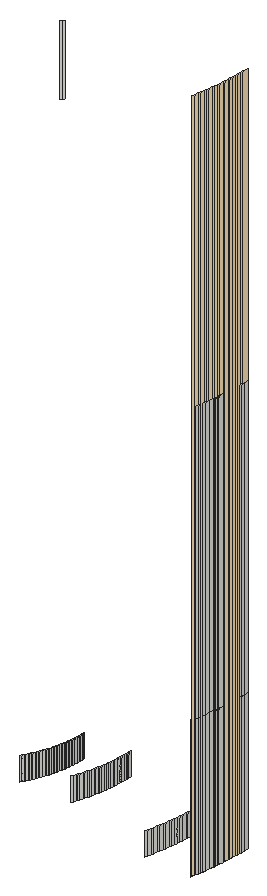
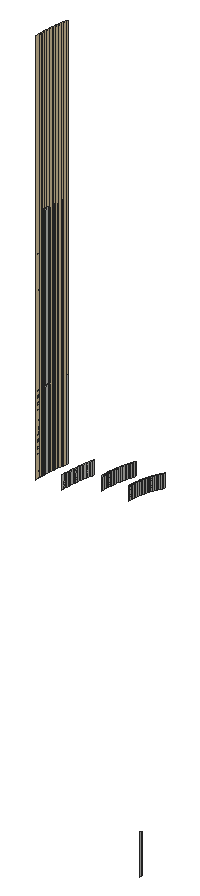
# SketchUp Ruby script. Lengths in inches.
U = 1.inch
M = Sketchup.active_model
def pt(a) = Geom::Point3d.new(a.map { |v| v * U })
def face(e, loops, mat)
  f = e.add_face(loops[0].map { |a| pt(a) })
  loops[1..].each { |l| e.add_face(l.map { |a| pt(a) }).erase! }
  f.material = f.back_material = mat if mat
  f
end
# faces: each face lists its corners as indices into pts; further lists are holes
def faces(e, pts, list, mat = nil) = list.each { |f| face(e, (f[0].is_a?(Array) ? f : [f]).map { |l| l.map { |i| pts[i] } }, mat) }
# xy, xz, yz: faces in a plane at the given z, y or x. An outline is a flat list of corners, or four numbers for a rectangle; further outlines are holes
def ring(l) = l.size == 4 ? [[l[0], l[1]], [l[2], l[1]], [l[2], l[3]], [l[0], l[3]]] : l.each_slice(2).to_a
def flat(e, list, mat, &to3) = list.each { |f| face(e, (f[0].is_a?(Array) ? f : [f]).map { |l| ring(l).map { |u, v| to3.(u, v) } }, mat) }
def xy(e, z, list, mat = nil) = flat(e, list, mat) { |x, y| [x, y, z] }
def xz(e, y, list, mat = nil) = flat(e, list, mat) { |x, z| [x, y, z] }
def yz(e, x, list, mat = nil) = flat(e, list, mat) { |y, z| [x, y, z] }
def lines(e, pts, list) = list.each { |a, b| e.add_line(pt(pts[a]), pt(pts[b])) }
# prism: a flat outline (further loops are holes) pulled along v
def prism(e, loops, v, mat = nil)
  f = face(e, loops, mat); d = Geom::Vector3d.new(v.map { |x| x * U })
  f.pushpull(f.normal.samedirection?(d) ? d.length : -d.length)
end
def box(e, o, s, mat = nil) = prism(e, [[o, [o[0] + s[0], o[1], o[2]], [o[0] + s[0], o[1] + s[1], o[2]], [o[0], o[1] + s[1], o[2]]]], [0, 0, s[2]], mat)
def at(x, y, z, deg = 0) = Geom::Transformation.translation(pt([x, y, z])) * Geom::Transformation.rotation(ORIGIN, Z_AXIS, deg.degrees)
def axes(o, x, y, z) = Geom::Transformation.new([*x, 0, *y, 0, *z, 0, *pt(o).to_a, 1])
def part(name) = M.definitions.add(name)
# library, detail: a bought-in or finely detailed component or shape, given as its bounding box
def library(name, o, s) = part(name).tap { |d| box(d.entities, o, s) }
def detail(e, o, s) = box(e.add_group.entities, o, s)
def put(e, d, t, mat = nil) = e.add_instance(d, t).tap { |i| i.material = mat if mat }
def group(e, t, mat = nil) = e.add_group.tap { |g| g.transformation = t; g.material = mat if mat }.entities
root = M.entities
M.materials.add("1026 AP 7946 SUNNY SIDE UP").color = [254, 231, 186]
yz(root,181.97,[[238.41,247,238.48,248]])
yz(root,181.98,[[238.54,247,238.61,248]])
yz(root,181.99,[[238.67,247,238.74,248]])
yz(root,182,[[238.8,247,238.87,248],[238.87,247,238.93,248],[238.93,247,239,248]])
yz(root,183.99,[[238.54,247,238.63,248],[238.63,247,238.73,248]])
yz(root,184,[[238.82,247,238.91,248],[238.91,247,239,248]])
yz(root,186.99,[[238.48,246,238.61,247]])
yz(root,187,[[238.74,246,238.87,247],[238.87,246,239,247]])
yz(root,188.98,[[238.25,246,238.37,276]],"1026 AP 7946 SUNNY SIDE UP")
yz(root,188.99,[[238.5,246,238.625,276]],"1026 AP 7946 SUNNY SIDE UP")
yz(root,189,[[238.6875,246,238.84,252],[238.84,246,239,252],[238.6875,252,238.84,264],[238.84,252,239,264]])
yz(root,189,[[238.75,246,239,276]],"1026 AP 7946 SUNNY SIDE UP")
p = [[186.69,236.54,246],[186.66,236.41,246],[186.66,236.41,247],[186.69,236.54,247],[188.74,236.51,252],[188.7,236.35,252],
  [188.7,236.35,246],[188.74,236.51,246],[188.74,236.51,246],[188.71,236.38,246],[188.71,236.38,276],[188.74,236.51,276],
  [186.72,236.67,246],[186.72,236.67,247],[188.77,236.66,252],[188.77,236.66,246],[188.76,236.63,246],[188.76,236.63,276],
  [188.79,236.75,246],[188.79,236.75,276],[186.75,236.79,246],[186.75,236.79,247],[188.8,236.8125,252],[188.8,236.8125,246],
  [186.78,236.92,246],[186.78,236.92,247],[188.83,236.97,252],[188.83,236.97,246],[188.81,236.875,246],[188.81,236.875,276],
  [186.81,237.05,246],[186.81,237.05,247],[188.83,237,246],[188.83,237,276],[186.83,237.18,246],[186.83,237.18,247],
  [188.85,237.12,252],[188.85,237.12,246],[188.85,237.12,246],[188.85,237.12,276],[188.875,237.28,252],[188.875,237.28,246],
  [188.87,237.25,246],[188.87,237.25,276],[186.86,237.31,246],[186.86,237.31,247],[188.89,237.37,246],[188.89,237.37,276],
  [186.875,237.4375,246],[186.875,237.4375,247],[188.9,237.43,252],[188.9,237.43,246],[186.9,237.57,246],[186.9,237.57,247],
  [188.92,237.59,252],[188.92,237.59,246],[188.91,237.5,246],[188.91,237.5,276],[188.92,237.62,246],[188.92,237.62,276],
  [186.91,237.69,246],[186.91,237.69,247],[188.93,237.75,252],[188.93,237.75,246],[188.93,237.75,246],[188.93,237.75,276],
  [186.93,237.82,246],[186.93,237.82,247],[188.95,237.9,252],[188.95,237.9,246],[188.95,237.87,246],[188.95,237.87,276],
  [186.95,237.95,246],[186.95,237.95,247],[188.96,238.06,252],[188.96,238.06,246],[188.96,238,246],[188.96,238,276],
  [186.96,238.08,246],[186.96,238.08,247],[188.97,238.12,246],[188.97,238.12,276],[186.97,238.22,246],[186.97,238.22,247],
  [188.97,238.22,252],[188.97,238.22,246],[188.98,238.25,246],[188.98,238.25,276],[186.98,238.35,246],[186.98,238.35,247],
  [188.98,238.37,252],[188.98,238.37,246],[186.99,238.48,246],[186.99,238.48,247],[188.99,238.53,252],[188.99,238.53,246],
  [188.99,238.5,246],[188.98,238.37,246],[188.98,238.37,276],[188.99,238.5,276],[189,238.6875,252],[189,238.6875,246],
  [187,238.74,246],[186.99,238.61,246],[186.99,238.61,247],[187,238.74,247],[189,238.75,246],[188.99,238.625,246],
  [188.99,238.625,276],[189,238.75,276],[181.3,236.44,247],[181.33,236.5,247],[181.33,236.5,248],[181.3,236.44,248],
  [183.54,236.49,248],[183.54,236.49,247],[183.5,236.41,247],[183.5,236.41,248],[181.36,236.56,247],[181.36,236.56,248],
  [183.57,236.58,248],[183.57,236.58,247],[181.39,236.61,247],[181.39,236.61,248],[181.42,236.67,247],[181.42,236.67,248],
  [183.6,236.66,248],[183.6,236.66,247],[181.46,236.73,247],[181.46,236.73,248],[181.48,236.79,247],[181.48,236.79,248],
  [183.63,236.75,248],[183.63,236.75,247],[183.66,236.84,248],[183.66,236.84,247],[181.51,236.85,247],[181.51,236.85,248],
  [181.54,236.91,247],[181.54,236.91,248],[183.69,236.92,248],[183.69,236.92,247],[181.57,236.97,247],[181.57,236.97,248],
  [183.71,237.01,248],[183.71,237.01,247],[181.59,237.03,247],[181.59,237.03,248],[181.62,237.09,247],[181.62,237.09,248],
  [183.74,237.1,248],[183.74,237.1,247],[181.64,237.15,247],[181.64,237.15,248],[181.67,237.21,247],[181.67,237.21,248],
  [183.76,237.1875,248],[183.76,237.1875,247],[181.69,237.27,247],[181.69,237.27,248],[183.78,237.28,248],[183.78,237.28,247],
  [181.71,237.33,247],[181.71,237.33,248],[181.73,237.39,247],[181.73,237.39,248],[183.81,237.37,248],[183.81,237.37,247],
  [181.76,237.45,247],[181.76,237.45,248],[183.83,237.46,248],[183.83,237.46,247],[181.78,237.52,247],[181.78,237.52,248],
  [181.79,237.58,247],[181.79,237.58,248],[183.85,237.54,248],[183.85,237.54,247],[183.87,237.63,248],[183.87,237.63,247],
  [181.8125,237.64,247],[181.8125,237.64,248],[181.83,237.71,247],[181.83,237.71,248],[183.88,237.72,248],[183.88,237.72,247],
  [181.85,237.77,247],[181.85,237.77,248],[183.9,237.81,248],[183.9,237.81,247],[181.86,237.83,247],[181.86,237.83,248],
  [181.875,237.9,247],[181.875,237.9,248],[183.91,237.9,248],[183.91,237.9,247],[181.89,237.96,247],[181.89,237.96,248],
  [183.93,238,248],[183.93,238,247],[181.9,238.02,247],[181.9,238.02,248],[181.92,238.09,247],[181.92,238.09,248],
  [183.94,238.09,248],[183.94,238.09,247],[181.93,238.15,247],[181.93,238.15,248],[183.95,238.18,248],[183.95,238.18,247],
  [181.9375,238.22,247],[181.9375,238.22,248],[181.95,238.28,247],[181.95,238.28,248],[183.96,238.27,248],[183.96,238.27,247],
  [181.96,238.35,247],[181.96,238.35,248],[181.97,238.41,247],[181.97,238.41,248],[183.97,238.36,248],[183.97,238.36,247],
  [183.98,238.45,248],[183.98,238.45,247],[181.97,238.48,247],[181.98,238.54,247],[181.98,238.54,248],[181.97,238.48,248],
  [183.99,238.54,248],[183.99,238.54,247],[181.98,238.61,247],[181.99,238.67,247],[181.99,238.67,248],[181.98,238.61,248],
  [181.99,238.74,247],[182,238.8,247],[182,238.8,248],[181.99,238.74,248],[184,238.82,248],[184,238.82,247],
  [183.99,238.73,247],[183.99,238.73,248],[153.23,273.8,250],[153.23,273.8,247],[153.17,273.74,247],[153.17,273.74,250],
  [153.28,273.86,250],[153.28,273.86,247],[188.77,236.66,264],[188.74,236.51,264],[188.74,236.51,252],[188.77,236.66,252],
  [188.8,236.8125,264],[188.8,236.8125,252],[188.83,236.97,264],[188.83,236.97,252],[188.85,237.12,264],[188.85,237.12,252],
  [188.875,237.28,264],[188.875,237.28,252],[188.9,237.43,264],[188.9,237.43,252],[188.92,237.59,264],[188.92,237.59,252],
  [188.93,237.75,264],[188.93,237.75,252],[188.95,237.9,264],[188.95,237.9,252],[188.96,238.06,264],[188.96,238.06,252],
  [188.97,238.22,264],[188.97,238.22,252],[188.98,238.37,264],[188.98,238.37,252],[188.99,238.53,264],[188.99,238.53,252],
  [189,238.6875,264],[189,238.6875,252],[186.95,239,246],[186.94,238.87,246],[186.94,238.74,246],[186.9375,238.61,246],
  [186.93,238.48,246],[186.92,238.35,246],[186.91,238.22,246],[186.9,238.09,246],[186.89,237.96,246],[186.875,237.83,246],
  [186.86,237.7,246],[186.84,237.57,246],[186.82,237.44,246],[186.8,237.32,246],[186.78,237.1875,246],[186.75,237.06,246],
  [186.73,236.93,246],[186.7,236.81,246],[186.67,236.68,246],[186.64,236.55,246],[186.61,236.43,246]]
faces(root,p,[[0,1,2,3],[4,5,6,7],[12,0,3,13],[14,4,7,15],[20,12,13,21],[22,14,15,23],[24,20,21,25],[26,22,23,27],
  [30,24,25,31],[34,30,31,35],[36,26,27,37],[40,36,37,41],[44,34,35,45],[48,44,45,49],[50,40,41,51],[52,48,49,53],
  [54,50,51,55],[60,52,53,61],[62,54,55,63],[66,60,61,67],[68,62,63,69],[72,66,67,73],[74,68,69,75],[78,72,73,79],
  [82,78,79,83],[84,74,75,85],[88,82,83,89],[90,84,85,91],[92,88,89,93],[94,90,91,95],[100,94,95,101],[102,103,104,105],
  [110,111,112,113],[114,115,116,117],[111,118,119,112],[120,121,115,114],[118,122,123,119],[122,124,125,123],[126,127,121,120],[124,128,129,125],
  [128,130,131,129],[132,133,127,126],[134,135,133,132],[130,136,137,131],[136,138,139,137],[140,141,135,134],[138,142,143,139],[144,145,141,140],
  [142,146,147,143],[146,148,149,147],[150,151,145,144],[148,152,153,149],[152,154,155,153],[156,157,151,150],[154,158,159,155],[160,161,157,156],
  [158,162,163,159],[162,164,165,163],[166,167,161,160],[164,168,169,165],[170,171,167,166],[168,172,173,169],[172,174,175,173],[176,177,171,170],
  [178,179,177,176],[174,180,181,175],[180,182,183,181],[184,185,179,178],[182,186,187,183],[188,189,185,184],[186,190,191,187],[190,192,193,191],
  [194,195,189,188],[192,196,197,193],[198,199,195,194],[196,200,201,197],[200,202,203,201],[204,205,199,198],[202,206,207,203],[208,209,205,204],
  [206,210,211,207],[210,212,213,211],[214,215,209,208],[212,216,217,213],[216,218,219,217],[220,221,215,214],[222,223,221,220],[224,225,226,227],
  [228,229,223,222],[230,231,232,233],[234,235,236,237],[238,239,240,241],[242,243,244,245],[246,247,243,242],[248,249,250,251],[252,248,251,253],
  [254,252,253,255],[256,254,255,257],[258,256,257,259],[260,258,259,261],[262,260,261,263],[264,262,263,265],[266,264,265,267],[268,266,267,269],
  [270,268,269,271],[272,270,271,273],[274,272,273,275],[276,274,275,277]])
faces(root,p,[[8,9,10,11],[16,8,11,17],[18,16,17,19],[28,18,19,29],[32,28,29,33],[38,32,33,39],[42,38,39,43],[46,42,43,47],
  [56,46,47,57],[58,56,57,59],[64,58,59,65],[70,64,65,71],[76,70,71,77],[80,76,77,81],[86,80,81,87],[96,97,98,99],
  [106,107,108,109]],"1026 AP 7946 SUNNY SIDE UP")
lines(root,p,[[278,279],[279,280],[280,281],[281,282],[282,283],[283,284],[284,285],[285,286],[286,287],[287,288],[288,289],[289,290],
  [290,291],[291,292],[292,293],[293,294],[294,295],[295,296],[296,297],[297,298]])
